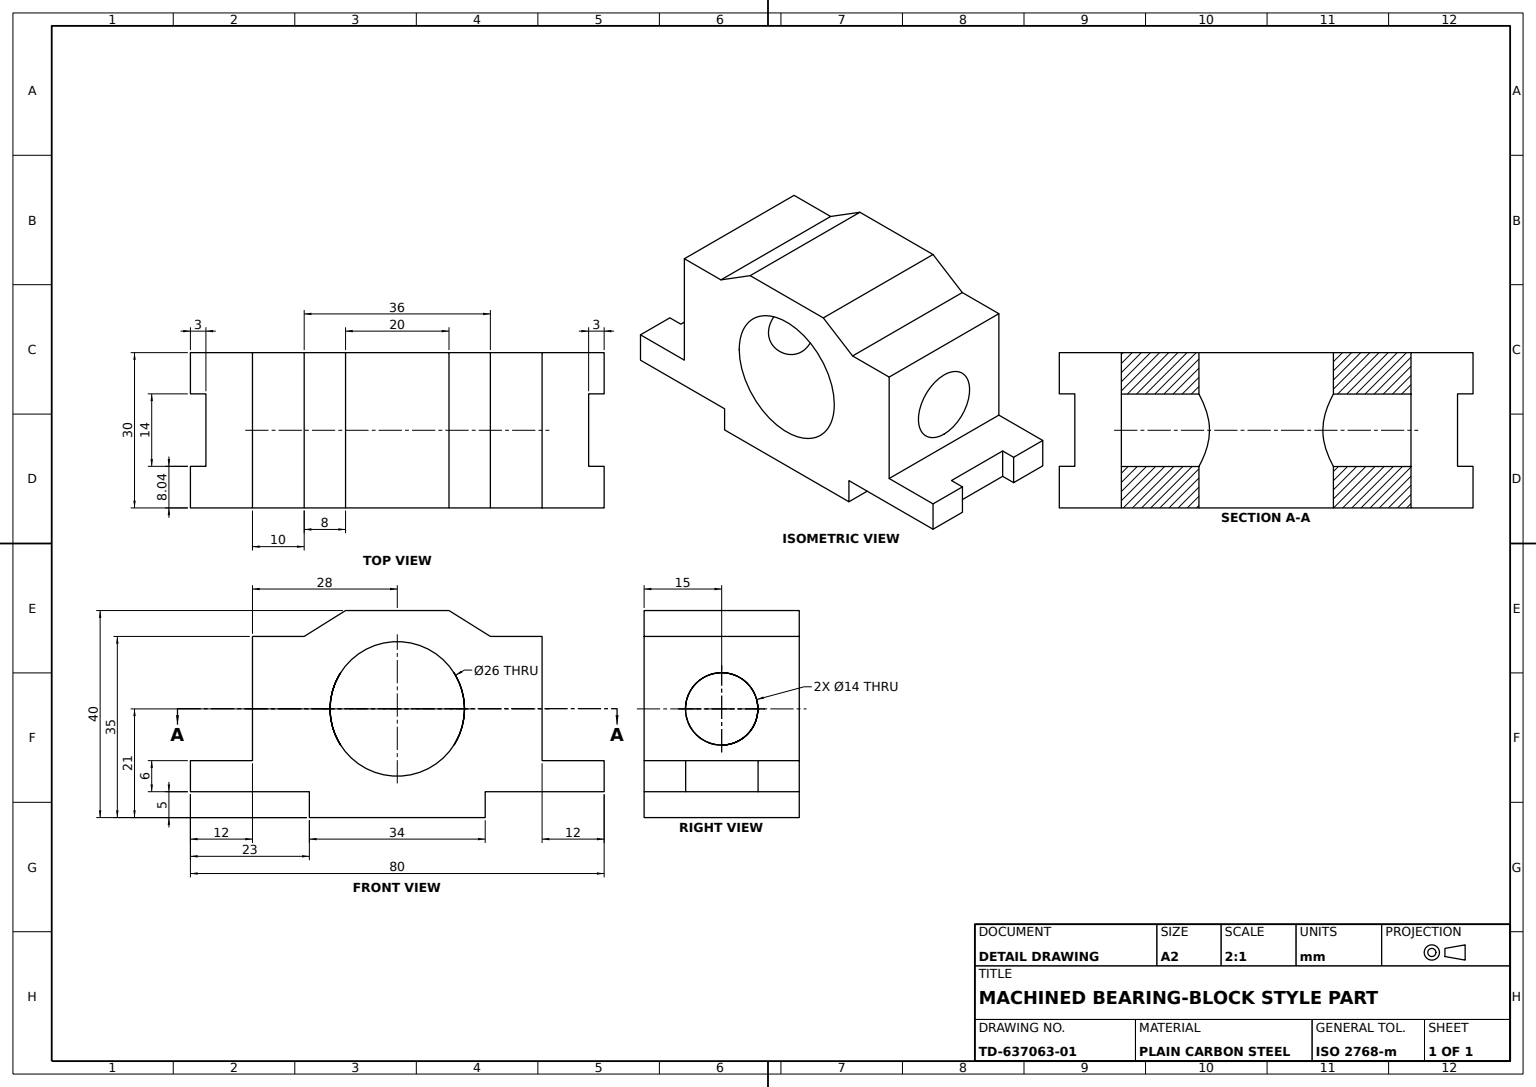
ISO-10303-21;
HEADER;
FILE_DESCRIPTION((''),'2;1');
FILE_NAME('','',(''),(''),'','','');
FILE_SCHEMA(('AUTOMOTIVE_DESIGN'));
ENDSEC;
DATA;
#1=APPLICATION_CONTEXT('');
#2=PRODUCT_CONTEXT('',#1,'mechanical');
#3=PRODUCT('','','',(#2));
#4=PRODUCT_DEFINITION_FORMATION('','',#3);
#5=PRODUCT_DEFINITION_CONTEXT('',#1,'design');
#6=PRODUCT_DEFINITION('','',#4,#5);
#7=PRODUCT_DEFINITION_SHAPE('','',#6);
#8=(LENGTH_UNIT()NAMED_UNIT(*)SI_UNIT(.MILLI.,.METRE.));
#9=(NAMED_UNIT(*)PLANE_ANGLE_UNIT()SI_UNIT($,.RADIAN.));
#10=(NAMED_UNIT(*)SI_UNIT($,.STERADIAN.)SOLID_ANGLE_UNIT());
#11=UNCERTAINTY_MEASURE_WITH_UNIT(LENGTH_MEASURE(1.E-05),#8,'distance_accuracy_value','');
#12=(GEOMETRIC_REPRESENTATION_CONTEXT(3)GLOBAL_UNCERTAINTY_ASSIGNED_CONTEXT((#11))GLOBAL_UNIT_ASSIGNED_CONTEXT((#8,#9,#10))REPRESENTATION_CONTEXT('',''));
#13=CARTESIAN_POINT('',(68.,6.,0.));
#14=VERTEX_POINT('',#13);
#15=CARTESIAN_POINT('',(68.,30.,0.));
#16=VERTEX_POINT('',#15);
#17=DIRECTION('',(0.,1.,0.));
#18=VECTOR('',#17,1000.);
#19=LINE('',#13,#18);
#20=EDGE_CURVE('',#14,#16,#19,.T.);
#21=ORIENTED_EDGE('',*,*,#20,.F.);
#22=CARTESIAN_POINT('',(68.,6.,-30.));
#23=VERTEX_POINT('',#22);
#24=DIRECTION('',(0.,0.,1.));
#25=VECTOR('',#24,1000.);
#26=LINE('',#22,#25);
#27=EDGE_CURVE('',#23,#14,#26,.T.);
#28=ORIENTED_EDGE('',*,*,#27,.F.);
#29=CARTESIAN_POINT('',(68.,30.,-30.));
#30=VERTEX_POINT('',#29);
#31=LINE('',#22,#18);
#32=EDGE_CURVE('',#23,#30,#31,.T.);
#33=ORIENTED_EDGE('',*,*,#32,.T.);
#34=LINE('',#29,#25);
#35=EDGE_CURVE('',#30,#16,#34,.T.);
#36=ORIENTED_EDGE('',*,*,#35,.T.);
#37=EDGE_LOOP('',(#21,#28,#33,#36));
#38=FACE_OUTER_BOUND('',#37,.T.);
#39=CARTESIAN_POINT('',(68.,23.,-15.));
#40=VERTEX_POINT('',#39);
#41=CARTESIAN_POINT('',(68.,9.,-15.));
#42=VERTEX_POINT('',#41);
#43=CARTESIAN_POINT('',(68.,16.,-15.));
#44=DIRECTION('',(1.,0.,0.));
#45=DIRECTION('',(0.,0.,-1.));
#46=AXIS2_PLACEMENT_3D('',#43,#44,#45);
#47=CIRCLE('',#46,7.);
#48=EDGE_CURVE('',#40,#42,#47,.T.);
#49=ORIENTED_EDGE('',*,*,#48,.F.);
#50=EDGE_CURVE('',#42,#40,#47,.T.);
#51=ORIENTED_EDGE('',*,*,#50,.F.);
#52=EDGE_LOOP('',(#49,#51));
#53=FACE_BOUND('',#52,.T.);
#54=AXIS2_PLACEMENT_3D('',#22,#44,#45);
#55=PLANE('',#54);
#56=ADVANCED_FACE('',(#38,#53),#55,.T.);
#57=CARTESIAN_POINT('',(57.,0.,0.));
#58=VERTEX_POINT('',#57);
#59=CARTESIAN_POINT('',(80.,0.,0.));
#60=VERTEX_POINT('',#59);
#61=VECTOR('',#44,1000.);
#62=LINE('',#57,#61);
#63=EDGE_CURVE('',#58,#60,#62,.T.);
#64=ORIENTED_EDGE('',*,*,#63,.F.);
#65=CARTESIAN_POINT('',(57.,0.,-30.));
#66=VERTEX_POINT('',#65);
#67=LINE('',#65,#25);
#68=EDGE_CURVE('',#66,#58,#67,.T.);
#69=ORIENTED_EDGE('',*,*,#68,.F.);
#70=CARTESIAN_POINT('',(80.,0.,-30.));
#71=VERTEX_POINT('',#70);
#72=LINE('',#65,#61);
#73=EDGE_CURVE('',#66,#71,#72,.T.);
#74=ORIENTED_EDGE('',*,*,#73,.T.);
#75=CARTESIAN_POINT('',(80.,0.,-22.037122));
#76=VERTEX_POINT('',#75);
#77=LINE('',#70,#25);
#78=EDGE_CURVE('',#71,#76,#77,.T.);
#79=ORIENTED_EDGE('',*,*,#78,.T.);
#80=CARTESIAN_POINT('',(77.,0.,-22.037122));
#81=VERTEX_POINT('',#80);
#82=CARTESIAN_POINT('',(57.,0.,-22.037122));
#83=LINE('',#82,#61);
#84=EDGE_CURVE('',#81,#76,#83,.T.);
#85=ORIENTED_EDGE('',*,*,#84,.F.);
#86=CARTESIAN_POINT('',(77.,0.,-8.037122));
#87=VERTEX_POINT('',#86);
#88=CARTESIAN_POINT('',(77.,0.,-30.));
#89=VECTOR('',#45,1000.);
#90=LINE('',#88,#89);
#91=EDGE_CURVE('',#87,#81,#90,.T.);
#92=ORIENTED_EDGE('',*,*,#91,.F.);
#93=CARTESIAN_POINT('',(80.,0.,-8.037122));
#94=VERTEX_POINT('',#93);
#95=CARTESIAN_POINT('',(57.,0.,-8.037122));
#96=DIRECTION('',(-1.,0.,0.));
#97=VECTOR('',#96,1000.);
#98=LINE('',#95,#97);
#99=EDGE_CURVE('',#94,#87,#98,.T.);
#100=ORIENTED_EDGE('',*,*,#99,.F.);
#101=EDGE_CURVE('',#94,#60,#77,.T.);
#102=ORIENTED_EDGE('',*,*,#101,.T.);
#103=EDGE_LOOP('',(#64,#69,#74,#79,#85,#92,#100,#102));
#104=FACE_OUTER_BOUND('',#103,.T.);
#105=DIRECTION('',(0.,-1.,0.));
#106=AXIS2_PLACEMENT_3D('',#65,#105,#45);
#107=PLANE('',#106);
#108=ADVANCED_FACE('',(#104),#107,.T.);
#109=CARTESIAN_POINT('',(12.,30.,0.));
#110=VERTEX_POINT('',#109);
#111=CARTESIAN_POINT('',(12.,6.,0.));
#112=VERTEX_POINT('',#111);
#113=VECTOR('',#105,1000.);
#114=LINE('',#109,#113);
#115=EDGE_CURVE('',#110,#112,#114,.T.);
#116=ORIENTED_EDGE('',*,*,#115,.F.);
#117=CARTESIAN_POINT('',(12.,30.,-30.));
#118=VERTEX_POINT('',#117);
#119=LINE('',#117,#25);
#120=EDGE_CURVE('',#118,#110,#119,.T.);
#121=ORIENTED_EDGE('',*,*,#120,.F.);
#122=CARTESIAN_POINT('',(12.,6.,-30.));
#123=VERTEX_POINT('',#122);
#124=LINE('',#117,#113);
#125=EDGE_CURVE('',#118,#123,#124,.T.);
#126=ORIENTED_EDGE('',*,*,#125,.T.);
#127=LINE('',#122,#25);
#128=EDGE_CURVE('',#123,#112,#127,.T.);
#129=ORIENTED_EDGE('',*,*,#128,.T.);
#130=EDGE_LOOP('',(#116,#121,#126,#129));
#131=FACE_OUTER_BOUND('',#130,.T.);
#132=CARTESIAN_POINT('',(12.,23.,-15.));
#133=VERTEX_POINT('',#132);
#134=CARTESIAN_POINT('',(12.,9.,-15.));
#135=VERTEX_POINT('',#134);
#136=CARTESIAN_POINT('',(12.,16.,-15.));
#137=AXIS2_PLACEMENT_3D('',#136,#96,#105);
#138=CIRCLE('',#137,7.);
#139=EDGE_CURVE('',#133,#135,#138,.T.);
#140=ORIENTED_EDGE('',*,*,#139,.F.);
#141=EDGE_CURVE('',#135,#133,#138,.T.);
#142=ORIENTED_EDGE('',*,*,#141,.F.);
#143=EDGE_LOOP('',(#140,#142));
#144=FACE_BOUND('',#143,.T.);
#145=AXIS2_PLACEMENT_3D('',#117,#96,#105);
#146=PLANE('',#145);
#147=ADVANCED_FACE('',(#131,#144),#146,.T.);
#148=CARTESIAN_POINT('',(0.,0.,-8.037122));
#149=VERTEX_POINT('',#148);
#150=CARTESIAN_POINT('',(0.,6.,-8.037122));
#151=VERTEX_POINT('',#150);
#152=CARTESIAN_POINT('',(0.,-5.,-8.037122));
#153=LINE('',#152,#18);
#154=EDGE_CURVE('',#149,#151,#153,.T.);
#155=ORIENTED_EDGE('',*,*,#154,.F.);
#156=CARTESIAN_POINT('',(0.,0.,0.));
#157=VERTEX_POINT('',#156);
#158=CARTESIAN_POINT('',(0.,0.,-30.));
#159=LINE('',#158,#25);
#160=EDGE_CURVE('',#149,#157,#159,.T.);
#161=ORIENTED_EDGE('',*,*,#160,.T.);
#162=CARTESIAN_POINT('',(0.,6.,0.));
#163=VERTEX_POINT('',#162);
#164=LINE('',#162,#113);
#165=EDGE_CURVE('',#163,#157,#164,.T.);
#166=ORIENTED_EDGE('',*,*,#165,.F.);
#167=CARTESIAN_POINT('',(0.,6.,-30.));
#168=LINE('',#167,#25);
#169=EDGE_CURVE('',#151,#163,#168,.T.);
#170=ORIENTED_EDGE('',*,*,#169,.F.);
#171=EDGE_LOOP('',(#155,#161,#166,#170));
#172=FACE_OUTER_BOUND('',#171,.T.);
#173=AXIS2_PLACEMENT_3D('',#167,#96,#105);
#174=PLANE('',#173);
#175=ADVANCED_FACE('',(#172),#174,.T.);
#176=CARTESIAN_POINT('',(30.,35.,-30.));
#177=VERTEX_POINT('',#176);
#178=CARTESIAN_POINT('',(30.,35.,0.));
#179=VERTEX_POINT('',#178);
#180=LINE('',#176,#25);
#181=EDGE_CURVE('',#177,#179,#180,.T.);
#182=ORIENTED_EDGE('',*,*,#181,.T.);
#183=CARTESIAN_POINT('',(50.,35.,0.));
#184=VERTEX_POINT('',#183);
#185=LINE('',#183,#97);
#186=EDGE_CURVE('',#184,#179,#185,.T.);
#187=ORIENTED_EDGE('',*,*,#186,.F.);
#188=CARTESIAN_POINT('',(50.,35.,-30.));
#189=VERTEX_POINT('',#188);
#190=LINE('',#188,#25);
#191=EDGE_CURVE('',#189,#184,#190,.T.);
#192=ORIENTED_EDGE('',*,*,#191,.F.);
#193=LINE('',#188,#97);
#194=EDGE_CURVE('',#189,#177,#193,.T.);
#195=ORIENTED_EDGE('',*,*,#194,.T.);
#196=EDGE_LOOP('',(#182,#187,#192,#195));
#197=FACE_OUTER_BOUND('',#196,.T.);
#198=AXIS2_PLACEMENT_3D('',#188,#17,#24);
#199=PLANE('',#198);
#200=ADVANCED_FACE('',(#197),#199,.T.);
#201=CARTESIAN_POINT('',(27.,16.,-30.));
#202=VERTEX_POINT('',#201);
#203=CARTESIAN_POINT('',(53.,16.,-30.));
#204=VERTEX_POINT('',#203);
#205=CARTESIAN_POINT('',(40.,16.,-30.));
#206=AXIS2_PLACEMENT_3D('',#205,#24,#44);
#207=CIRCLE('',#206,13.);
#208=EDGE_CURVE('',#202,#204,#207,.T.);
#209=ORIENTED_EDGE('',*,*,#208,.T.);
#210=EDGE_CURVE('',#204,#202,#207,.T.);
#211=ORIENTED_EDGE('',*,*,#210,.T.);
#212=EDGE_LOOP('',(#209,#211));
#213=FACE_BOUND('',#212,.T.);
#214=CARTESIAN_POINT('',(58.,30.,-30.));
#215=VERTEX_POINT('',#214);
#216=LINE('',#29,#97);
#217=EDGE_CURVE('',#30,#215,#216,.T.);
#218=ORIENTED_EDGE('',*,*,#217,.F.);
#219=ORIENTED_EDGE('',*,*,#32,.F.);
#220=CARTESIAN_POINT('',(80.,6.,-30.));
#221=VERTEX_POINT('',#220);
#222=LINE('',#220,#97);
#223=EDGE_CURVE('',#221,#23,#222,.T.);
#224=ORIENTED_EDGE('',*,*,#223,.F.);
#225=LINE('',#70,#18);
#226=EDGE_CURVE('',#71,#221,#225,.T.);
#227=ORIENTED_EDGE('',*,*,#226,.F.);
#228=ORIENTED_EDGE('',*,*,#73,.F.);
#229=CARTESIAN_POINT('',(57.,-5.,-30.));
#230=VERTEX_POINT('',#229);
#231=LINE('',#229,#18);
#232=EDGE_CURVE('',#230,#66,#231,.T.);
#233=ORIENTED_EDGE('',*,*,#232,.F.);
#234=CARTESIAN_POINT('',(23.,-5.,-30.));
#235=VERTEX_POINT('',#234);
#236=LINE('',#234,#61);
#237=EDGE_CURVE('',#235,#230,#236,.T.);
#238=ORIENTED_EDGE('',*,*,#237,.F.);
#239=CARTESIAN_POINT('',(23.,0.,-30.));
#240=VERTEX_POINT('',#239);
#241=LINE('',#239,#113);
#242=EDGE_CURVE('',#240,#235,#241,.T.);
#243=ORIENTED_EDGE('',*,*,#242,.F.);
#244=VERTEX_POINT('',#158);
#245=LINE('',#158,#61);
#246=EDGE_CURVE('',#244,#240,#245,.T.);
#247=ORIENTED_EDGE('',*,*,#246,.F.);
#248=VERTEX_POINT('',#167);
#249=LINE('',#167,#113);
#250=EDGE_CURVE('',#248,#244,#249,.T.);
#251=ORIENTED_EDGE('',*,*,#250,.F.);
#252=LINE('',#122,#97);
#253=EDGE_CURVE('',#123,#248,#252,.T.);
#254=ORIENTED_EDGE('',*,*,#253,.F.);
#255=ORIENTED_EDGE('',*,*,#125,.F.);
#256=CARTESIAN_POINT('',(22.,30.,-30.));
#257=VERTEX_POINT('',#256);
#258=LINE('',#256,#97);
#259=EDGE_CURVE('',#257,#118,#258,.T.);
#260=ORIENTED_EDGE('',*,*,#259,.F.);
#261=DIRECTION('',(-0.847998304,-0.52999894,0.));
#262=VECTOR('',#261,1000.);
#263=LINE('',#176,#262);
#264=EDGE_CURVE('',#177,#257,#263,.T.);
#265=ORIENTED_EDGE('',*,*,#264,.F.);
#266=ORIENTED_EDGE('',*,*,#194,.F.);
#267=DIRECTION('',(-0.847998304,0.52999894,0.));
#268=VECTOR('',#267,1000.);
#269=LINE('',#214,#268);
#270=EDGE_CURVE('',#215,#189,#269,.T.);
#271=ORIENTED_EDGE('',*,*,#270,.F.);
#272=EDGE_LOOP('',(#218,#219,#224,#227,#228,#233,#238,#243,#247,#251,#254,#255,#260,#265,#266,#271));
#273=FACE_OUTER_BOUND('',#272,.T.);
#274=AXIS2_PLACEMENT_3D('',#158,#24,#44);
#275=PLANE('',#274);
#276=ADVANCED_FACE('',(#213,#273),#275,.F.);
#277=ORIENTED_EDGE('',*,*,#120,.T.);
#278=CARTESIAN_POINT('',(22.,30.,0.));
#279=VERTEX_POINT('',#278);
#280=LINE('',#278,#97);
#281=EDGE_CURVE('',#279,#110,#280,.T.);
#282=ORIENTED_EDGE('',*,*,#281,.F.);
#283=LINE('',#256,#25);
#284=EDGE_CURVE('',#257,#279,#283,.T.);
#285=ORIENTED_EDGE('',*,*,#284,.F.);
#286=ORIENTED_EDGE('',*,*,#259,.T.);
#287=EDGE_LOOP('',(#277,#282,#285,#286));
#288=FACE_OUTER_BOUND('',#287,.T.);
#289=AXIS2_PLACEMENT_3D('',#256,#17,#96);
#290=PLANE('',#289);
#291=ADVANCED_FACE('',(#288),#290,.T.);
#292=CARTESIAN_POINT('',(80.,6.,-22.037122));
#293=VERTEX_POINT('',#292);
#294=CARTESIAN_POINT('',(77.,6.,-22.037122));
#295=VERTEX_POINT('',#294);
#296=LINE('',#292,#97);
#297=EDGE_CURVE('',#293,#295,#296,.T.);
#298=ORIENTED_EDGE('',*,*,#297,.T.);
#299=CARTESIAN_POINT('',(77.,-5.,-22.037122));
#300=LINE('',#299,#18);
#301=EDGE_CURVE('',#81,#295,#300,.T.);
#302=ORIENTED_EDGE('',*,*,#301,.F.);
#303=ORIENTED_EDGE('',*,*,#84,.T.);
#304=CARTESIAN_POINT('',(80.,-5.,-22.037122));
#305=LINE('',#304,#18);
#306=EDGE_CURVE('',#76,#293,#305,.T.);
#307=ORIENTED_EDGE('',*,*,#306,.T.);
#308=EDGE_LOOP('',(#298,#302,#303,#307));
#309=FACE_OUTER_BOUND('',#308,.T.);
#310=AXIS2_PLACEMENT_3D('',#304,#45,#96);
#311=PLANE('',#310);
#312=ADVANCED_FACE('',(#309),#311,.F.);
#313=CARTESIAN_POINT('',(80.,6.,0.));
#314=VERTEX_POINT('',#313);
#315=LINE('',#59,#18);
#316=EDGE_CURVE('',#60,#314,#315,.T.);
#317=ORIENTED_EDGE('',*,*,#316,.F.);
#318=ORIENTED_EDGE('',*,*,#101,.F.);
#319=CARTESIAN_POINT('',(80.,6.,-8.037122));
#320=VERTEX_POINT('',#319);
#321=CARTESIAN_POINT('',(80.,-5.,-8.037122));
#322=LINE('',#321,#18);
#323=EDGE_CURVE('',#94,#320,#322,.T.);
#324=ORIENTED_EDGE('',*,*,#323,.T.);
#325=LINE('',#220,#25);
#326=EDGE_CURVE('',#320,#314,#325,.T.);
#327=ORIENTED_EDGE('',*,*,#326,.T.);
#328=EDGE_LOOP('',(#317,#318,#324,#327));
#329=FACE_OUTER_BOUND('',#328,.T.);
#330=AXIS2_PLACEMENT_3D('',#70,#44,#45);
#331=PLANE('',#330);
#332=ADVANCED_FACE('',(#329),#331,.T.);
#333=CARTESIAN_POINT('',(3.,6.,-22.037122));
#334=VERTEX_POINT('',#333);
#335=CARTESIAN_POINT('',(0.,6.,-22.037122));
#336=VERTEX_POINT('',#335);
#337=LINE('',#335,#97);
#338=EDGE_CURVE('',#334,#336,#337,.T.);
#339=ORIENTED_EDGE('',*,*,#338,.F.);
#340=CARTESIAN_POINT('',(3.,6.,-8.037122));
#341=VERTEX_POINT('',#340);
#342=LINE('',#333,#89);
#343=EDGE_CURVE('',#341,#334,#342,.T.);
#344=ORIENTED_EDGE('',*,*,#343,.F.);
#345=LINE('',#340,#61);
#346=EDGE_CURVE('',#151,#341,#345,.T.);
#347=ORIENTED_EDGE('',*,*,#346,.F.);
#348=ORIENTED_EDGE('',*,*,#169,.T.);
#349=LINE('',#111,#97);
#350=EDGE_CURVE('',#112,#163,#349,.T.);
#351=ORIENTED_EDGE('',*,*,#350,.F.);
#352=ORIENTED_EDGE('',*,*,#128,.F.);
#353=ORIENTED_EDGE('',*,*,#253,.T.);
#354=EDGE_CURVE('',#248,#336,#168,.T.);
#355=ORIENTED_EDGE('',*,*,#354,.T.);
#356=EDGE_LOOP('',(#339,#344,#347,#348,#351,#352,#353,#355));
#357=FACE_OUTER_BOUND('',#356,.T.);
#358=AXIS2_PLACEMENT_3D('',#122,#17,#96);
#359=PLANE('',#358);
#360=ADVANCED_FACE('',(#357),#359,.T.);
#361=ORIENTED_EDGE('',*,*,#208,.F.);
#362=CARTESIAN_POINT('',(27.,16.,-22.));
#363=VERTEX_POINT('',#362);
#364=LINE('',#201,#25);
#365=EDGE_CURVE('',#202,#363,#364,.T.);
#366=ORIENTED_EDGE('',*,*,#365,.T.);
#367=CARTESIAN_POINT('',(29.045549,9.,-15.));
#368=VERTEX_POINT('',#367);
#369=CARTESIAN_POINT('',(27.,15.535136,-22.));
#370=CARTESIAN_POINT('',(27.025824,15.061814,-21.952365));
#371=CARTESIAN_POINT('',(27.123913,14.15181,-21.767552));
#372=CARTESIAN_POINT('',(27.195579,13.711673,-21.631518));
#373=CARTESIAN_POINT('',(27.377421,12.859913,-21.273223));
#374=CARTESIAN_POINT('',(27.48536,12.459138,-21.055242));
#375=CARTESIAN_POINT('',(27.721655,11.710925,-20.55045));
#376=CARTESIAN_POINT('',(27.851721,11.359239,-20.259708));
#377=CARTESIAN_POINT('',(28.112987,10.725887,-19.624384));
#378=CARTESIAN_POINT('',(28.244552,10.442267,-19.279556));
#379=CARTESIAN_POINT('',(28.432901,10.065191,-18.718708));
#380=CARTESIAN_POINT('',(28.494491,9.947046,-18.523257));
#381=CARTESIAN_POINT('',(28.61056,9.731375,-18.123449));
#382=CARTESIAN_POINT('',(28.665093,9.633676,-17.919117));
#383=CARTESIAN_POINT('',(28.815595,9.370525,-17.292459));
#384=CARTESIAN_POINT('',(28.898562,9.234638,-16.856633));
#385=CARTESIAN_POINT('',(28.985394,9.094823,-16.171677));
#386=CARTESIAN_POINT('',(29.00791,9.059198,-15.938268));
#387=CARTESIAN_POINT('',(29.037894,9.011938,-15.471251));
#388=CARTESIAN_POINT('',(29.045549,9.,-15.235728));
#389=B_SPLINE_CURVE_WITH_KNOTS('',3,(#362,#369,#370,#371,#372,#373,#374,#375,#376,#377,#378,#379,#380,#381,#382,#383,#384,#385,#386,#387,#388,#367),.UNSPECIFIED.,.F.,.F.,(4,2,2,2,2,2,2,2,2,2,4),(0.033482105,0.03487358,0.036265056,0.037656532,0.039048007,0.040439483,0.041135221,0.041830959,0.043222435,0.043918172,0.04461391),.UNSPECIFIED.);
#390=EDGE_CURVE('',#363,#368,#389,.T.);
#391=ORIENTED_EDGE('',*,*,#390,.T.);
#392=CARTESIAN_POINT('',(27.,16.,-8.));
#393=VERTEX_POINT('',#392);
#394=CARTESIAN_POINT('',(29.045549,9.,-14.526856));
#395=CARTESIAN_POINT('',(29.014841,9.047449,-14.064004));
#396=CARTESIAN_POINT('',(28.900724,9.231117,-13.1571));
#397=CARTESIAN_POINT('',(28.816001,9.369789,-12.708976));
#398=CARTESIAN_POINT('',(28.613683,9.72359,-11.867083));
#399=CARTESIAN_POINT('',(28.496083,9.93864,-11.469291));
#400=CARTESIAN_POINT('',(28.243054,10.445325,-10.716126));
#401=CARTESIAN_POINT('',(28.110311,10.731936,-10.368796));
#402=CARTESIAN_POINT('',(27.914713,11.206762,-9.893631));
#403=CARTESIAN_POINT('',(27.849952,11.372828,-9.742599));
#404=CARTESIAN_POINT('',(27.722911,11.721277,-9.455316));
#405=CARTESIAN_POINT('',(27.660391,11.904521,-9.318588));
#406=CARTESIAN_POINT('',(27.482563,12.468805,-8.938958));
#407=CARTESIAN_POINT('',(27.375891,12.86675,-8.723745));
#408=CARTESIAN_POINT('',(27.241149,13.498389,-8.45828));
#409=CARTESIAN_POINT('',(27.200448,13.714762,-8.379428));
#410=CARTESIAN_POINT('',(27.128889,14.160065,-8.242121));
#411=CARTESIAN_POINT('',(27.098434,14.386949,-8.184434));
#412=CARTESIAN_POINT('',(27.025276,15.069447,-8.046617));
#413=CARTESIAN_POINT('',(27.,15.531208,-8.));
#414=B_SPLINE_CURVE_WITH_KNOTS('',3,(#367,#394,#395,#396,#397,#398,#399,#400,#401,#402,#403,#404,#405,#406,#407,#408,#409,#410,#411,#412,#413,#392),.UNSPECIFIED.,.F.,.F.,(4,2,2,2,2,2,2,2,2,2,4),(0.,0.001396458,0.002792916,0.004189374,0.005585831,0.00628406,0.006982289,0.008378747,0.009076976,0.009775205,0.011171663),.UNSPECIFIED.);
#415=EDGE_CURVE('',#368,#393,#414,.T.);
#416=ORIENTED_EDGE('',*,*,#415,.T.);
#417=CARTESIAN_POINT('',(27.,16.,0.));
#418=VERTEX_POINT('',#417);
#419=EDGE_CURVE('',#393,#418,#364,.T.);
#420=ORIENTED_EDGE('',*,*,#419,.T.);
#421=CARTESIAN_POINT('',(53.,16.,0.));
#422=VERTEX_POINT('',#421);
#423=CARTESIAN_POINT('',(40.,16.,0.));
#424=AXIS2_PLACEMENT_3D('',#423,#24,#44);
#425=CIRCLE('',#424,13.);
#426=EDGE_CURVE('',#418,#422,#425,.T.);
#427=ORIENTED_EDGE('',*,*,#426,.T.);
#428=CARTESIAN_POINT('',(53.,16.,-8.));
#429=VERTEX_POINT('',#428);
#430=LINE('',#203,#25);
#431=EDGE_CURVE('',#429,#422,#430,.T.);
#432=ORIENTED_EDGE('',*,*,#431,.F.);
#433=CARTESIAN_POINT('',(50.954451,9.,-15.));
#434=VERTEX_POINT('',#433);
#435=CARTESIAN_POINT('',(53.,15.766756,-8.));
#436=CARTESIAN_POINT('',(52.993651,15.530991,-8.01177));
#437=CARTESIAN_POINT('',(52.968301,15.062928,-8.059018));
#438=CARTESIAN_POINT('',(52.949474,14.832365,-8.094176));
#439=CARTESIAN_POINT('',(52.900421,14.377841,-8.186603));
#440=CARTESIAN_POINT('',(52.870192,14.153882,-8.243875));
#441=CARTESIAN_POINT('',(52.7991,13.712418,-8.380306));
#442=CARTESIAN_POINT('',(52.758019,13.493936,-8.459892));
#443=CARTESIAN_POINT('',(52.621423,12.855281,-8.729096));
#444=CARTESIAN_POINT('',(52.513846,12.456233,-8.94637));
#445=CARTESIAN_POINT('',(52.276787,11.706387,-9.452963));
#446=CARTESIAN_POINT('',(52.146469,11.354547,-9.744475));
#447=CARTESIAN_POINT('',(51.885437,10.722374,-10.379671));
#448=CARTESIAN_POINT('',(51.753602,10.438311,-10.725331));
#449=CARTESIAN_POINT('',(51.564392,10.059905,-11.289667));
#450=CARTESIAN_POINT('',(51.502946,9.942192,-11.485152));
#451=CARTESIAN_POINT('',(51.387485,9.727839,-11.88372));
#452=CARTESIAN_POINT('',(51.33313,9.630515,-12.087782));
#453=CARTESIAN_POINT('',(51.18289,9.367985,-12.714878));
#454=CARTESIAN_POINT('',(51.099517,9.231494,-13.154208));
#455=CARTESIAN_POINT('',(50.984163,9.045856,-14.072906));
#456=CARTESIAN_POINT('',(50.954451,9.,-14.535054));
#457=B_SPLINE_CURVE_WITH_KNOTS('',3,(#428,#435,#436,#437,#438,#439,#440,#441,#442,#443,#444,#445,#446,#447,#448,#449,#450,#451,#452,#453,#454,#455,#456,#433),.UNSPECIFIED.,.F.,.F.,(4,2,2,2,2,2,2,2,2,2,2,4),(0.022336639,0.023033746,0.023730854,0.024427961,0.025125069,0.026519283,0.027913498,0.029307713,0.030004821,0.030701928,0.032096143,0.033490358),.UNSPECIFIED.);
#458=EDGE_CURVE('',#429,#434,#457,.T.);
#459=ORIENTED_EDGE('',*,*,#458,.T.);
#460=CARTESIAN_POINT('',(53.,16.,-22.));
#461=VERTEX_POINT('',#460);
#462=CARTESIAN_POINT('',(50.954451,9.,-15.232022));
#463=CARTESIAN_POINT('',(50.96183,9.011505,-15.464744));
#464=CARTESIAN_POINT('',(50.991526,9.058306,-15.931626));
#465=CARTESIAN_POINT('',(51.013842,9.093609,-16.164274));
#466=CARTESIAN_POINT('',(51.099753,9.231894,-16.846027));
#467=CARTESIAN_POINT('',(51.182598,9.367386,-17.284752));
#468=CARTESIAN_POINT('',(51.386274,9.723469,-18.13318));
#469=CARTESIAN_POINT('',(51.504259,9.939417,-18.531515));
#470=CARTESIAN_POINT('',(51.754913,10.441164,-19.278037));
#471=CARTESIAN_POINT('',(51.889052,10.73049,-19.629583));
#472=CARTESIAN_POINT('',(52.150012,11.363783,-20.263675));
#473=CARTESIAN_POINT('',(52.277544,11.708547,-20.548706));
#474=CARTESIAN_POINT('',(52.455266,12.271057,-20.92842));
#475=CARTESIAN_POINT('',(52.512548,12.4674,-21.047548));
#476=CARTESIAN_POINT('',(52.619006,12.868896,-21.264846));
#477=CARTESIAN_POINT('',(52.668289,13.074167,-21.36328));
#478=CARTESIAN_POINT('',(52.80278,13.703696,-21.628298));
#479=CARTESIAN_POINT('',(52.874715,14.141526,-21.764952));
#480=CARTESIAN_POINT('',(52.97397,15.057498,-21.951992));
#481=CARTESIAN_POINT('',(53.,15.528903,-22.));
#482=B_SPLINE_CURVE_WITH_KNOTS('',3,(#433,#462,#463,#464,#465,#466,#467,#468,#469,#470,#471,#472,#473,#474,#475,#476,#477,#478,#479,#480,#481,#460),.UNSPECIFIED.,.F.,.F.,(4,2,2,2,2,2,2,2,2,2,4),(0.033490358,0.034186112,0.034881865,0.036273373,0.037664881,0.039056389,0.040447897,0.041143651,0.041839405,0.043230912,0.04462242),.UNSPECIFIED.);
#483=EDGE_CURVE('',#434,#461,#482,.T.);
#484=ORIENTED_EDGE('',*,*,#483,.T.);
#485=EDGE_CURVE('',#204,#461,#430,.T.);
#486=ORIENTED_EDGE('',*,*,#485,.F.);
#487=EDGE_LOOP('',(#361,#366,#391,#416,#420,#427,#432,#459,#484,#486));
#488=FACE_OUTER_BOUND('',#487,.T.);
#489=CYLINDRICAL_SURFACE('',#206,13.);
#490=ADVANCED_FACE('',(#488),#489,.F.);
#491=CARTESIAN_POINT('',(3.,0.,-22.037122));
#492=VERTEX_POINT('',#491);
#493=CARTESIAN_POINT('',(3.,-5.,-22.037122));
#494=LINE('',#493,#18);
#495=EDGE_CURVE('',#492,#334,#494,.T.);
#496=ORIENTED_EDGE('',*,*,#495,.F.);
#497=CARTESIAN_POINT('',(3.,0.,-8.037122));
#498=VERTEX_POINT('',#497);
#499=CARTESIAN_POINT('',(3.,0.,-30.));
#500=LINE('',#499,#25);
#501=EDGE_CURVE('',#492,#498,#500,.T.);
#502=ORIENTED_EDGE('',*,*,#501,.T.);
#503=CARTESIAN_POINT('',(3.,-5.,-8.037122));
#504=LINE('',#503,#18);
#505=EDGE_CURVE('',#498,#341,#504,.T.);
#506=ORIENTED_EDGE('',*,*,#505,.T.);
#507=ORIENTED_EDGE('',*,*,#343,.T.);
#508=EDGE_LOOP('',(#496,#502,#506,#507));
#509=FACE_OUTER_BOUND('',#508,.T.);
#510=AXIS2_PLACEMENT_3D('',#493,#44,#17);
#511=PLANE('',#510);
#512=ADVANCED_FACE('',(#509),#511,.F.);
#513=EDGE_CURVE('',#221,#293,#325,.T.);
#514=ORIENTED_EDGE('',*,*,#513,.T.);
#515=ORIENTED_EDGE('',*,*,#306,.F.);
#516=ORIENTED_EDGE('',*,*,#78,.F.);
#517=ORIENTED_EDGE('',*,*,#226,.T.);
#518=EDGE_LOOP('',(#514,#515,#516,#517));
#519=FACE_OUTER_BOUND('',#518,.T.);
#520=ADVANCED_FACE('',(#519),#331,.T.);
#521=CARTESIAN_POINT('',(57.,-5.,0.));
#522=VERTEX_POINT('',#521);
#523=LINE('',#229,#25);
#524=EDGE_CURVE('',#230,#522,#523,.T.);
#525=ORIENTED_EDGE('',*,*,#524,.T.);
#526=CARTESIAN_POINT('',(23.,-5.,0.));
#527=VERTEX_POINT('',#526);
#528=LINE('',#526,#61);
#529=EDGE_CURVE('',#527,#522,#528,.T.);
#530=ORIENTED_EDGE('',*,*,#529,.F.);
#531=LINE('',#234,#25);
#532=EDGE_CURVE('',#235,#527,#531,.T.);
#533=ORIENTED_EDGE('',*,*,#532,.F.);
#534=ORIENTED_EDGE('',*,*,#237,.T.);
#535=EDGE_LOOP('',(#525,#530,#533,#534));
#536=FACE_OUTER_BOUND('',#535,.T.);
#537=AXIS2_PLACEMENT_3D('',#234,#105,#45);
#538=PLANE('',#537);
#539=ADVANCED_FACE('',(#536),#538,.T.);
#540=LINE('',#148,#97);
#541=EDGE_CURVE('',#498,#149,#540,.T.);
#542=ORIENTED_EDGE('',*,*,#541,.F.);
#543=ORIENTED_EDGE('',*,*,#501,.F.);
#544=CARTESIAN_POINT('',(0.,0.,-22.037122));
#545=VERTEX_POINT('',#544);
#546=LINE('',#544,#61);
#547=EDGE_CURVE('',#545,#492,#546,.T.);
#548=ORIENTED_EDGE('',*,*,#547,.F.);
#549=EDGE_CURVE('',#244,#545,#159,.T.);
#550=ORIENTED_EDGE('',*,*,#549,.F.);
#551=ORIENTED_EDGE('',*,*,#246,.T.);
#552=CARTESIAN_POINT('',(23.,0.,0.));
#553=VERTEX_POINT('',#552);
#554=LINE('',#239,#25);
#555=EDGE_CURVE('',#240,#553,#554,.T.);
#556=ORIENTED_EDGE('',*,*,#555,.T.);
#557=LINE('',#156,#61);
#558=EDGE_CURVE('',#157,#553,#557,.T.);
#559=ORIENTED_EDGE('',*,*,#558,.F.);
#560=ORIENTED_EDGE('',*,*,#160,.F.);
#561=EDGE_LOOP('',(#542,#543,#548,#550,#551,#556,#559,#560));
#562=FACE_OUTER_BOUND('',#561,.T.);
#563=AXIS2_PLACEMENT_3D('',#158,#105,#45);
#564=PLANE('',#563);
#565=ADVANCED_FACE('',(#562),#564,.T.);
#566=ORIENTED_EDGE('',*,*,#50,.T.);
#567=CARTESIAN_POINT('',(50.954451,23.,-15.));
#568=VERTEX_POINT('',#567);
#569=CARTESIAN_POINT('',(80.,23.,-15.));
#570=LINE('',#569,#97);
#571=EDGE_CURVE('',#40,#568,#570,.T.);
#572=ORIENTED_EDGE('',*,*,#571,.T.);
#573=CARTESIAN_POINT('',(53.,16.472989,-22.));
#574=CARTESIAN_POINT('',(52.974286,16.936394,-21.952567));
#575=CARTESIAN_POINT('',(52.87648,17.845315,-21.768296));
#576=CARTESIAN_POINT('',(52.803088,18.295192,-21.628924));
#577=CARTESIAN_POINT('',(52.622274,19.140888,-21.272588));
#578=CARTESIAN_POINT('',(52.514909,19.540297,-21.05588));
#579=CARTESIAN_POINT('',(52.335993,20.106392,-20.67357));
#580=CARTESIAN_POINT('',(52.273583,20.288744,-20.536916));
#581=CARTESIAN_POINT('',(52.146706,20.635912,-20.249674));
#582=CARTESIAN_POINT('',(52.08197,20.801587,-20.098523));
#583=CARTESIAN_POINT('',(51.951493,21.117719,-19.781121));
#584=CARTESIAN_POINT('',(51.885748,21.268177,-19.614872));
#585=CARTESIAN_POINT('',(51.754929,21.553947,-19.266661));
#586=CARTESIAN_POINT('',(51.689578,21.689774,-19.083809));
#587=CARTESIAN_POINT('',(51.500921,22.066949,-18.520827));
#588=CARTESIAN_POINT('',(51.38404,22.280495,-18.124445));
#589=CARTESIAN_POINT('',(51.233226,22.544073,-17.495357));
#590=CARTESIAN_POINT('',(51.187057,22.622394,-17.279863));
#591=CARTESIAN_POINT('',(51.105131,22.758876,-16.836158));
#592=CARTESIAN_POINT('',(51.069803,22.81633,-16.609732));
#593=CARTESIAN_POINT('',(50.984535,22.95353,-15.928877));
#594=CARTESIAN_POINT('',(50.954451,23.,-15.468082));
#595=B_SPLINE_CURVE_WITH_KNOTS('',3,(#460,#573,#574,#575,#576,#577,#578,#579,#580,#581,#582,#583,#584,#585,#586,#587,#588,#589,#590,#591,#592,#593,#594,#567),.UNSPECIFIED.,.F.,.F.,(4,2,2,2,2,2,2,2,2,2,2,4),(0.,0.001397096,0.002794193,0.004191289,0.004889838,0.005588386,0.006286934,0.006985482,0.008382579,0.009081127,0.009779675,0.011176772),.UNSPECIFIED.);
#596=EDGE_CURVE('',#461,#568,#595,.T.);
#597=ORIENTED_EDGE('',*,*,#596,.F.);
#598=ORIENTED_EDGE('',*,*,#483,.F.);
#599=CARTESIAN_POINT('',(80.,9.,-15.));
#600=LINE('',#599,#97);
#601=EDGE_CURVE('',#42,#434,#600,.T.);
#602=ORIENTED_EDGE('',*,*,#601,.F.);
#603=EDGE_LOOP('',(#566,#572,#597,#598,#602));
#604=FACE_OUTER_BOUND('',#603,.T.);
#605=CARTESIAN_POINT('',(80.,16.,-15.));
#606=AXIS2_PLACEMENT_3D('',#605,#96,#105);
#607=CYLINDRICAL_SURFACE('',#606,7.);
#608=ADVANCED_FACE('',(#604),#607,.F.);
#609=EDGE_CURVE('',#422,#418,#425,.T.);
#610=ORIENTED_EDGE('',*,*,#609,.T.);
#611=ORIENTED_EDGE('',*,*,#419,.F.);
#612=CARTESIAN_POINT('',(29.045549,23.,-15.));
#613=VERTEX_POINT('',#612);
#614=CARTESIAN_POINT('',(27.,16.234183,-8.));
#615=CARTESIAN_POINT('',(27.006453,16.471355,-8.011964));
#616=CARTESIAN_POINT('',(27.031733,16.937268,-8.059081));
#617=CARTESIAN_POINT('',(27.050493,17.16724,-8.094114));
#618=CARTESIAN_POINT('',(27.099492,17.621438,-8.186437));
#619=CARTESIAN_POINT('',(27.129732,17.845664,-8.243727));
#620=CARTESIAN_POINT('',(27.201041,18.288436,-8.380578));
#621=CARTESIAN_POINT('',(27.24235,18.507872,-8.460614));
#622=CARTESIAN_POINT('',(27.378497,19.144176,-8.728947));
#623=CARTESIAN_POINT('',(27.485965,19.54321,-8.945955));
#624=CARTESIAN_POINT('',(27.664238,20.107047,-9.326939));
#625=CARTESIAN_POINT('',(27.726799,20.289853,-9.463922));
#626=CARTESIAN_POINT('',(27.854,20.637779,-9.751952));
#627=CARTESIAN_POINT('',(27.918805,20.803531,-9.903315));
#628=CARTESIAN_POINT('',(28.114424,21.277295,-10.379327));
#629=CARTESIAN_POINT('',(28.24691,21.562794,-10.726664));
#630=CARTESIAN_POINT('',(28.499674,22.06814,-11.480944));
#631=CARTESIAN_POINT('',(28.616597,22.28163,-11.878005));
#632=CARTESIAN_POINT('',(28.766972,22.544407,-12.505573));
#633=CARTESIAN_POINT('',(28.812914,22.622339,-12.720133));
#634=CARTESIAN_POINT('',(28.894353,22.758023,-13.160897));
#635=CARTESIAN_POINT('',(28.929983,22.815985,-13.388638));
#636=CARTESIAN_POINT('',(29.015712,22.95393,-14.072943));
#637=CARTESIAN_POINT('',(29.045549,23.,-14.533985));
#638=B_SPLINE_CURVE_WITH_KNOTS('',3,(#392,#614,#615,#616,#617,#618,#619,#620,#621,#622,#623,#624,#625,#626,#627,#628,#629,#630,#631,#632,#633,#634,#635,#636,#637,#612),.UNSPECIFIED.,.F.,.F.,(4,2,2,2,2,2,2,2,2,2,2,2,4),(0.011171663,0.011869257,0.012566852,0.013264447,0.013962041,0.015357231,0.016054825,0.01675242,0.018147609,0.019542799,0.020240393,0.020937988,0.022333177),.UNSPECIFIED.);
#639=EDGE_CURVE('',#393,#613,#638,.T.);
#640=ORIENTED_EDGE('',*,*,#639,.T.);
#641=CARTESIAN_POINT('',(29.045549,23.,-15.46549));
#642=CARTESIAN_POINT('',(29.014544,22.952089,-15.939672));
#643=CARTESIAN_POINT('',(28.928622,22.813775,-16.620525));
#644=CARTESIAN_POINT('',(28.893544,22.756694,-16.84394));
#645=CARTESIAN_POINT('',(28.812065,22.620904,-17.283998));
#646=CARTESIAN_POINT('',(28.765413,22.541758,-17.501642));
#647=CARTESIAN_POINT('',(28.612624,22.274535,-18.137105));
#648=CARTESIAN_POINT('',(28.494866,22.058968,-18.534437));
#649=CARTESIAN_POINT('',(28.243437,21.555397,-19.282629));
#650=CARTESIAN_POINT('',(28.109256,21.265686,-19.633895));
#651=CARTESIAN_POINT('',(27.848555,20.632452,-20.266956));
#652=CARTESIAN_POINT('',(27.72076,20.286825,-20.55249));
#653=CARTESIAN_POINT('',(27.542251,19.720705,-20.933642));
#654=CARTESIAN_POINT('',(27.485174,19.524482,-21.052249));
#655=CARTESIAN_POINT('',(27.37932,19.124305,-21.268207));
#656=CARTESIAN_POINT('',(27.330214,18.919348,-21.366258));
#657=CARTESIAN_POINT('',(27.196003,18.289534,-21.630641));
#658=CARTESIAN_POINT('',(27.123679,17.847744,-21.768002));
#659=CARTESIAN_POINT('',(27.024942,16.928258,-21.954017));
#660=CARTESIAN_POINT('',(27.,16.465579,-22.));
#661=B_SPLINE_CURVE_WITH_KNOTS('',3,(#612,#641,#642,#643,#644,#645,#646,#647,#648,#649,#650,#651,#652,#653,#654,#655,#656,#657,#658,#659,#660,#362),.UNSPECIFIED.,.F.,.F.,(4,2,2,2,2,2,2,2,2,2,4),(0.022333177,0.023726793,0.024423601,0.025120409,0.026514025,0.027907641,0.029301257,0.029998065,0.030694873,0.032088489,0.033482105),.UNSPECIFIED.);
#662=EDGE_CURVE('',#613,#363,#661,.T.);
#663=ORIENTED_EDGE('',*,*,#662,.T.);
#664=ORIENTED_EDGE('',*,*,#365,.F.);
#665=ORIENTED_EDGE('',*,*,#210,.F.);
#666=ORIENTED_EDGE('',*,*,#485,.T.);
#667=ORIENTED_EDGE('',*,*,#596,.T.);
#668=CARTESIAN_POINT('',(50.954451,23.,-14.766313));
#669=CARTESIAN_POINT('',(50.962097,22.988076,-14.529183));
#670=CARTESIAN_POINT('',(50.991985,22.940969,-14.063081));
#671=CARTESIAN_POINT('',(51.014111,22.905961,-13.83329));
#672=CARTESIAN_POINT('',(51.071324,22.813863,-13.379879));
#673=CARTESIAN_POINT('',(51.106411,22.75677,-13.156261));
#674=CARTESIAN_POINT('',(51.188128,22.620581,-12.715001));
#675=CARTESIAN_POINT('',(51.234992,22.541057,-12.496596));
#676=CARTESIAN_POINT('',(51.387319,22.274618,-11.863285));
#677=CARTESIAN_POINT('',(51.505003,22.059254,-11.465895));
#678=CARTESIAN_POINT('',(51.694107,21.680474,-10.903254));
#679=CARTESIAN_POINT('',(51.759452,21.544372,-10.720914));
#680=CARTESIAN_POINT('',(51.890211,21.258102,-10.373663));
#681=CARTESIAN_POINT('',(51.955888,21.107448,-10.207921));
#682=CARTESIAN_POINT('',(52.151294,20.632833,-9.733402));
#683=CARTESIAN_POINT('',(52.279891,20.285021,-9.446065));
#684=CARTESIAN_POINT('',(52.518147,19.528899,-8.937453));
#685=CARTESIAN_POINT('',(52.624823,19.130233,-8.722321));
#686=CARTESIAN_POINT('',(52.759148,18.500055,-8.457704));
#687=CARTESIAN_POINT('',(52.799641,18.284596,-8.379259));
#688=CARTESIAN_POINT('',(52.870764,17.842178,-8.242784));
#689=CARTESIAN_POINT('',(52.901478,17.613894,-8.184601));
#690=CARTESIAN_POINT('',(52.974936,16.928538,-8.046218));
#691=CARTESIAN_POINT('',(53.,16.466746,-8.));
#692=B_SPLINE_CURVE_WITH_KNOTS('',3,(#567,#668,#669,#670,#671,#672,#673,#674,#675,#676,#677,#678,#679,#680,#681,#682,#683,#684,#685,#686,#687,#688,#689,#690,#691,#428),.UNSPECIFIED.,.F.,.F.,(4,2,2,2,2,2,2,2,2,2,2,2,4),(0.011176772,0.011874264,0.012571755,0.013269247,0.013966739,0.015361722,0.016059214,0.016756705,0.018151689,0.019546672,0.020244164,0.020941656,0.022336639),.UNSPECIFIED.);
#693=EDGE_CURVE('',#568,#429,#692,.T.);
#694=ORIENTED_EDGE('',*,*,#693,.T.);
#695=ORIENTED_EDGE('',*,*,#431,.T.);
#696=EDGE_LOOP('',(#610,#611,#640,#663,#664,#665,#666,#667,#694,#695));
#697=FACE_OUTER_BOUND('',#696,.T.);
#698=ADVANCED_FACE('',(#697),#489,.F.);
#699=ORIENTED_EDGE('',*,*,#505,.F.);
#700=ORIENTED_EDGE('',*,*,#541,.T.);
#701=ORIENTED_EDGE('',*,*,#154,.T.);
#702=ORIENTED_EDGE('',*,*,#346,.T.);
#703=EDGE_LOOP('',(#699,#700,#701,#702));
#704=FACE_OUTER_BOUND('',#703,.T.);
#705=AXIS2_PLACEMENT_3D('',#503,#24,#44);
#706=PLANE('',#705);
#707=ADVANCED_FACE('',(#704),#706,.F.);
#708=ORIENTED_EDGE('',*,*,#693,.F.);
#709=ORIENTED_EDGE('',*,*,#571,.F.);
#710=ORIENTED_EDGE('',*,*,#48,.T.);
#711=ORIENTED_EDGE('',*,*,#601,.T.);
#712=ORIENTED_EDGE('',*,*,#458,.F.);
#713=EDGE_LOOP('',(#708,#709,#710,#711,#712));
#714=FACE_OUTER_BOUND('',#713,.T.);
#715=ADVANCED_FACE('',(#714),#607,.F.);
#716=CARTESIAN_POINT('',(77.,6.,-8.037122));
#717=VERTEX_POINT('',#716);
#718=LINE('',#716,#61);
#719=EDGE_CURVE('',#717,#320,#718,.T.);
#720=ORIENTED_EDGE('',*,*,#719,.T.);
#721=ORIENTED_EDGE('',*,*,#323,.F.);
#722=ORIENTED_EDGE('',*,*,#99,.T.);
#723=CARTESIAN_POINT('',(77.,-5.,-8.037122));
#724=LINE('',#723,#18);
#725=EDGE_CURVE('',#87,#717,#724,.T.);
#726=ORIENTED_EDGE('',*,*,#725,.T.);
#727=EDGE_LOOP('',(#720,#721,#722,#726));
#728=FACE_OUTER_BOUND('',#727,.T.);
#729=AXIS2_PLACEMENT_3D('',#723,#24,#44);
#730=PLANE('',#729);
#731=ADVANCED_FACE('',(#728),#730,.F.);
#732=ORIENTED_EDGE('',*,*,#242,.T.);
#733=ORIENTED_EDGE('',*,*,#532,.T.);
#734=LINE('',#552,#113);
#735=EDGE_CURVE('',#553,#527,#734,.T.);
#736=ORIENTED_EDGE('',*,*,#735,.F.);
#737=ORIENTED_EDGE('',*,*,#555,.F.);
#738=EDGE_LOOP('',(#732,#733,#736,#737));
#739=FACE_OUTER_BOUND('',#738,.T.);
#740=AXIS2_PLACEMENT_3D('',#239,#96,#24);
#741=PLANE('',#740);
#742=ADVANCED_FACE('',(#739),#741,.T.);
#743=ORIENTED_EDGE('',*,*,#415,.F.);
#744=EDGE_CURVE('',#368,#135,#600,.T.);
#745=ORIENTED_EDGE('',*,*,#744,.T.);
#746=ORIENTED_EDGE('',*,*,#141,.T.);
#747=EDGE_CURVE('',#613,#133,#570,.T.);
#748=ORIENTED_EDGE('',*,*,#747,.F.);
#749=ORIENTED_EDGE('',*,*,#639,.F.);
#750=EDGE_LOOP('',(#743,#745,#746,#748,#749));
#751=FACE_OUTER_BOUND('',#750,.T.);
#752=ADVANCED_FACE('',(#751),#607,.F.);
#753=ORIENTED_EDGE('',*,*,#232,.T.);
#754=ORIENTED_EDGE('',*,*,#68,.T.);
#755=LINE('',#521,#18);
#756=EDGE_CURVE('',#522,#58,#755,.T.);
#757=ORIENTED_EDGE('',*,*,#756,.F.);
#758=ORIENTED_EDGE('',*,*,#524,.F.);
#759=EDGE_LOOP('',(#753,#754,#757,#758));
#760=FACE_OUTER_BOUND('',#759,.T.);
#761=AXIS2_PLACEMENT_3D('',#229,#44,#45);
#762=PLANE('',#761);
#763=ADVANCED_FACE('',(#760),#762,.T.);
#764=ORIENTED_EDGE('',*,*,#297,.F.);
#765=ORIENTED_EDGE('',*,*,#513,.F.);
#766=ORIENTED_EDGE('',*,*,#223,.T.);
#767=ORIENTED_EDGE('',*,*,#27,.T.);
#768=LINE('',#313,#97);
#769=EDGE_CURVE('',#314,#14,#768,.T.);
#770=ORIENTED_EDGE('',*,*,#769,.F.);
#771=ORIENTED_EDGE('',*,*,#326,.F.);
#772=ORIENTED_EDGE('',*,*,#719,.F.);
#773=LINE('',#294,#25);
#774=EDGE_CURVE('',#295,#717,#773,.T.);
#775=ORIENTED_EDGE('',*,*,#774,.F.);
#776=EDGE_LOOP('',(#764,#765,#766,#767,#770,#771,#772,#775));
#777=FACE_OUTER_BOUND('',#776,.T.);
#778=AXIS2_PLACEMENT_3D('',#220,#17,#96);
#779=PLANE('',#778);
#780=ADVANCED_FACE('',(#777),#779,.T.);
#781=ORIENTED_EDGE('',*,*,#20,.T.);
#782=CARTESIAN_POINT('',(58.,30.,0.));
#783=VERTEX_POINT('',#782);
#784=LINE('',#15,#97);
#785=EDGE_CURVE('',#16,#783,#784,.T.);
#786=ORIENTED_EDGE('',*,*,#785,.T.);
#787=LINE('',#782,#268);
#788=EDGE_CURVE('',#783,#184,#787,.T.);
#789=ORIENTED_EDGE('',*,*,#788,.T.);
#790=ORIENTED_EDGE('',*,*,#186,.T.);
#791=LINE('',#178,#262);
#792=EDGE_CURVE('',#179,#279,#791,.T.);
#793=ORIENTED_EDGE('',*,*,#792,.T.);
#794=ORIENTED_EDGE('',*,*,#281,.T.);
#795=ORIENTED_EDGE('',*,*,#115,.T.);
#796=ORIENTED_EDGE('',*,*,#350,.T.);
#797=ORIENTED_EDGE('',*,*,#165,.T.);
#798=ORIENTED_EDGE('',*,*,#558,.T.);
#799=ORIENTED_EDGE('',*,*,#735,.T.);
#800=ORIENTED_EDGE('',*,*,#529,.T.);
#801=ORIENTED_EDGE('',*,*,#756,.T.);
#802=ORIENTED_EDGE('',*,*,#63,.T.);
#803=ORIENTED_EDGE('',*,*,#316,.T.);
#804=ORIENTED_EDGE('',*,*,#769,.T.);
#805=EDGE_LOOP('',(#781,#786,#789,#790,#793,#794,#795,#796,#797,#798,#799,#800,#801,#802,#803,#804));
#806=FACE_OUTER_BOUND('',#805,.T.);
#807=ORIENTED_EDGE('',*,*,#609,.F.);
#808=ORIENTED_EDGE('',*,*,#426,.F.);
#809=EDGE_LOOP('',(#807,#808));
#810=FACE_BOUND('',#809,.T.);
#811=AXIS2_PLACEMENT_3D('',#156,#24,#44);
#812=PLANE('',#811);
#813=ADVANCED_FACE('',(#806,#810),#812,.T.);
#814=ORIENTED_EDGE('',*,*,#284,.T.);
#815=ORIENTED_EDGE('',*,*,#792,.F.);
#816=ORIENTED_EDGE('',*,*,#181,.F.);
#817=ORIENTED_EDGE('',*,*,#264,.T.);
#818=EDGE_LOOP('',(#814,#815,#816,#817));
#819=FACE_OUTER_BOUND('',#818,.T.);
#820=DIRECTION('',(-0.52999894,0.847998304,0.));
#821=AXIS2_PLACEMENT_3D('',#176,#820,#261);
#822=PLANE('',#821);
#823=ADVANCED_FACE('',(#819),#822,.T.);
#824=CARTESIAN_POINT('',(0.,-5.,-22.037122));
#825=LINE('',#824,#18);
#826=EDGE_CURVE('',#545,#336,#825,.T.);
#827=ORIENTED_EDGE('',*,*,#826,.T.);
#828=ORIENTED_EDGE('',*,*,#354,.F.);
#829=ORIENTED_EDGE('',*,*,#250,.T.);
#830=ORIENTED_EDGE('',*,*,#549,.T.);
#831=EDGE_LOOP('',(#827,#828,#829,#830));
#832=FACE_OUTER_BOUND('',#831,.T.);
#833=ADVANCED_FACE('',(#832),#174,.T.);
#834=ORIENTED_EDGE('',*,*,#747,.T.);
#835=ORIENTED_EDGE('',*,*,#139,.T.);
#836=ORIENTED_EDGE('',*,*,#744,.F.);
#837=ORIENTED_EDGE('',*,*,#390,.F.);
#838=ORIENTED_EDGE('',*,*,#662,.F.);
#839=EDGE_LOOP('',(#834,#835,#836,#837,#838));
#840=FACE_OUTER_BOUND('',#839,.T.);
#841=ADVANCED_FACE('',(#840),#607,.F.);
#842=ORIENTED_EDGE('',*,*,#826,.F.);
#843=ORIENTED_EDGE('',*,*,#547,.T.);
#844=ORIENTED_EDGE('',*,*,#495,.T.);
#845=ORIENTED_EDGE('',*,*,#338,.T.);
#846=EDGE_LOOP('',(#842,#843,#844,#845));
#847=FACE_OUTER_BOUND('',#846,.T.);
#848=AXIS2_PLACEMENT_3D('',#824,#45,#96);
#849=PLANE('',#848);
#850=ADVANCED_FACE('',(#847),#849,.F.);
#851=ORIENTED_EDGE('',*,*,#35,.F.);
#852=ORIENTED_EDGE('',*,*,#217,.T.);
#853=LINE('',#214,#25);
#854=EDGE_CURVE('',#215,#783,#853,.T.);
#855=ORIENTED_EDGE('',*,*,#854,.T.);
#856=ORIENTED_EDGE('',*,*,#785,.F.);
#857=EDGE_LOOP('',(#851,#852,#855,#856));
#858=FACE_OUTER_BOUND('',#857,.T.);
#859=AXIS2_PLACEMENT_3D('',#29,#17,#24);
#860=PLANE('',#859);
#861=ADVANCED_FACE('',(#858),#860,.T.);
#862=ORIENTED_EDGE('',*,*,#270,.T.);
#863=ORIENTED_EDGE('',*,*,#191,.T.);
#864=ORIENTED_EDGE('',*,*,#788,.F.);
#865=ORIENTED_EDGE('',*,*,#854,.F.);
#866=EDGE_LOOP('',(#862,#863,#864,#865));
#867=FACE_OUTER_BOUND('',#866,.T.);
#868=DIRECTION('',(0.52999894,0.847998304,0.));
#869=AXIS2_PLACEMENT_3D('',#214,#868,#267);
#870=PLANE('',#869);
#871=ADVANCED_FACE('',(#867),#870,.T.);
#872=ORIENTED_EDGE('',*,*,#301,.T.);
#873=ORIENTED_EDGE('',*,*,#774,.T.);
#874=ORIENTED_EDGE('',*,*,#725,.F.);
#875=ORIENTED_EDGE('',*,*,#91,.T.);
#876=EDGE_LOOP('',(#872,#873,#874,#875));
#877=FACE_OUTER_BOUND('',#876,.T.);
#878=AXIS2_PLACEMENT_3D('',#299,#96,#24);
#879=PLANE('',#878);
#880=ADVANCED_FACE('',(#877),#879,.F.);
#881=CLOSED_SHELL('',(#56,#108,#147,#175,#200,#276,#291,#312,#332,#360,#490,#512,#520,#539,#565,#608,#698,#707,#715,#731,#742,#752,#763,#780,#813,#823,#833,#841,#850,#861,#871,#880));
#882=MANIFOLD_SOLID_BREP('',#881);
#883=ADVANCED_BREP_SHAPE_REPRESENTATION('',(#882),#12);
#884=SHAPE_DEFINITION_REPRESENTATION(#7,#883);
ENDSEC;
END-ISO-10303-21;
